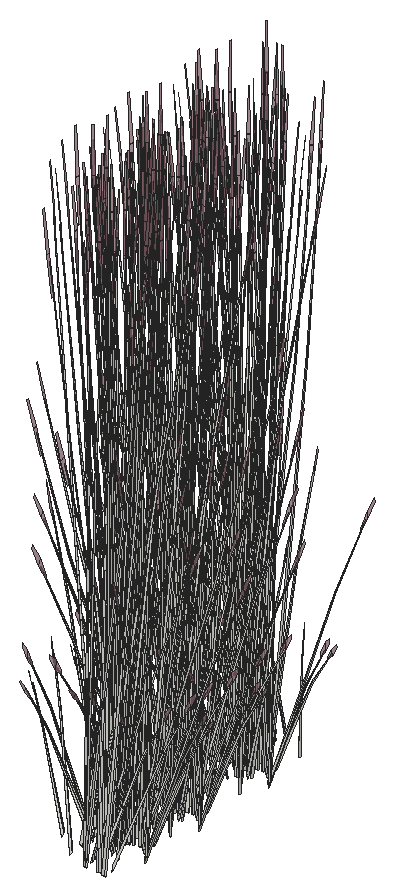
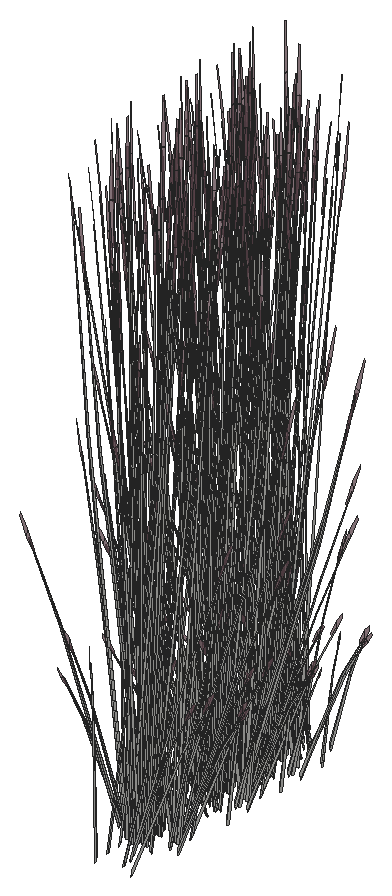
# SketchUp Ruby script. Lengths in inches.
U = 1.inch
M = Sketchup.active_model
def pt(a) = Geom::Point3d.new(a.map { |v| v * U })
def face(e, loops, mat)
  f = e.add_face(loops[0].map { |a| pt(a) })
  loops[1..].each { |l| e.add_face(l.map { |a| pt(a) }).erase! }
  f.material = f.back_material = mat if mat
  f
end
# faces: each face lists its corners as indices into pts; further lists are holes
def faces(e, pts, list, mat = nil) = list.each { |f| face(e, (f[0].is_a?(Array) ? f : [f]).map { |l| l.map { |i| pts[i] } }, mat) }
# xy, xz, yz: faces in a plane at the given z, y or x. An outline is a flat list of corners, or four numbers for a rectangle; further outlines are holes
def ring(l) = l.size == 4 ? [[l[0], l[1]], [l[2], l[1]], [l[2], l[3]], [l[0], l[3]]] : l.each_slice(2).to_a
def flat(e, list, mat, &to3) = list.each { |f| face(e, (f[0].is_a?(Array) ? f : [f]).map { |l| ring(l).map { |u, v| to3.(u, v) } }, mat) }
def xy(e, z, list, mat = nil) = flat(e, list, mat) { |x, y| [x, y, z] }
def xz(e, y, list, mat = nil) = flat(e, list, mat) { |x, z| [x, y, z] }
def yz(e, x, list, mat = nil) = flat(e, list, mat) { |y, z| [x, y, z] }
def lines(e, pts, list) = list.each { |a, b| e.add_line(pt(pts[a]), pt(pts[b])) }
# prism: a flat outline (further loops are holes) pulled along v
def prism(e, loops, v, mat = nil)
  f = face(e, loops, mat); d = Geom::Vector3d.new(v.map { |x| x * U })
  f.pushpull(f.normal.samedirection?(d) ? d.length : -d.length)
end
def box(e, o, s, mat = nil) = prism(e, [[o, [o[0] + s[0], o[1], o[2]], [o[0] + s[0], o[1] + s[1], o[2]], [o[0], o[1] + s[1], o[2]]]], [0, 0, s[2]], mat)
def at(x, y, z, deg = 0) = Geom::Transformation.translation(pt([x, y, z])) * Geom::Transformation.rotation(ORIGIN, Z_AXIS, deg.degrees)
def axes(o, x, y, z) = Geom::Transformation.new([*x, 0, *y, 0, *z, 0, *pt(o).to_a, 1])
def part(name) = M.definitions.add(name)
# library, detail: a bought-in or finely detailed component or shape, given as its bounding box
def library(name, o, s) = part(name).tap { |d| box(d.entities, o, s) }
def detail(e, o, s) = box(e.add_group.entities, o, s)
def put(e, d, t, mat = nil) = e.add_instance(d, t).tap { |i| i.material = mat if mat }
def group(e, t, mat = nil) = e.add_group.tap { |g| g.transformation = t; g.material = mat if mat }.entities
root = M.entities
M.materials.add("LightPink_Translucent").color = [144, 107, 117]
M.materials["LightPink_Translucent"].alpha = 0.75
c1 = part("blade")
p = [[2.15,0.21,22],[0,0.17,0],[0.09,0.45,0],[2.18,0.31,22],[2.29,0.31,22],[0.38,0.45,0],
  [2.48,0.24,33],[2.49,0.24,33],[2.48,0.22,33]]
faces(c1.entities,p,[[0,1,2,3],[4,5,2,3],[6,3,4,7],[8,0,3,6]])
c2 = part("seeds")
p = [[0.3,-0.1,1.38],[-0.01,-0.03,1.59],[-0.01,-0.03,0.03],[0.14,-0.07,-0.07],[0.29,-0.03,3],[0.15,0.01,3.11]]
faces(c2.entities,p,[[0,1,2,3],[1,0,4,5]],"LightPink_Translucent")
c3 = part("blade with seeds")
put(c3.entities,c1,at(0,0,0))
put(c3.entities,c2,axes([2.4,0.25,30.99],[1.5799,-0.05474,1.17369],[-0.12525,1.92788,0.29478],[-0.07173,-0.02425,1.56792]))
put(root,c3,axes([431.12,469.63,152.01],[0.51243,0,0],[0,0.52715,-0.43598],[0,0.12006,1.38303]))
put(root,c3,axes([430.91,469.9,151.86],[-0.51218,-0.00377,-0.04204],[0,-0.52715,0.42192],[-0.0161,0.12,1.33776]))
put(root,c3,axes([429.8,469.44,152.25],[0.46151,0.22505,-0.2458],[-0.22222,0.475,-0.42242],[0.0145,0.11662,1.34921]))
put(root,c3,axes([427.74,473.58,151.97],[-0.38118,0.39654,0.25983],[-0.38142,-0.39237,-0.30828],[-0.01331,-0.11261,1.39295]))
put(root,c3,axes([426.58,471.19,152.34],[0.17079,-0.21377,0.97034],[0.06739,0.33841,0.71294],[-0.12342,0.0606,0.21373]))
put(root,c3,axes([429.57,470.01,152.25],[0.04775,0.53819,-0.2458],[-0.49736,0.03254,-0.42242],[-0.08758,0.07169,1.34921]))
put(root,c3,axes([428.95,473.77,152.06],[0.46174,0.2286,0.2033],[-0.22222,0.475,0.42242],[0,-0.1095,1.35626]))
put(root,c3,axes([428.77,474.41,152.06],[0.10862,-0.55889,-0.19793],[0.515,0.09742,0.43313],[-0.08999,-0.07718,1.32161]))
put(root,c3,axes([426.95,473.17,152.34],[0.26163,-0.03375,0.97034],[-0.16596,0.29737,0.71294],[-0.12929,-0.04461,0.21373]))
put(root,c3,axes([428.8,473.45,152.3],[-0.44501,0.02912,0.37796],[-0.04024,-0.48332,-0.1819],[0.07967,-0.04899,1.2135]))
put(root,c3,axes([427.65,473.8,152.09],[0,0.47166,0.41945],[-0.45849,0,0],[0,-0.10742,1.33059]))
put(root,c3,axes([429.76,471.02,151.97],[0.51304,0.1533,0.25983],[-0.12835,0.54797,-0.30828],[-0.08491,0.06858,1.39295]))
put(root,c3,axes([430.27,472.16,152.01],[0.25622,-0.47263,0],[0.42866,0.26357,-0.43598],[0.09763,0.06003,1.38303]))
put(root,c3,axes([428.79,473.62,151.99],[0.17817,0.52741,0.38653],[-0.50909,0.1834,0.15168],[0.00622,-0.09691,1.34202]))
put(root,c3,axes([431.28,474.03,151.67],[-0.26394,0.0566,1.1961],[-0.04201,-0.45055,0.06846],[0.18486,-0.06819,0.68062]))
put(root,c3,axes([431.76,473.625,151.91],[-0.25407,-0.3016,-0.05481],[0.27826,-0.27635,-0.2485],[0.07884,-0.01946,0.81966]))
put(root,c3,axes([428.7,474.04,152.3],[-0.19883,0.425,0.37796],[-0.41314,-0.20454,-0.1819],[0,-0.09797,1.2135]))
put(root,c3,axes([430.42,470.97,152.34],[-0.23074,-0.13562,0.97034],[0.29794,-0.1378,0.71294],[0.08036,0.11673,0.21373]))
put(root,c3,axes([429.43,473.67,151.86],[0,-0.54574,0],[0.51243,0,0],[0,0,1.51605]))
put(root,c3,axes([430.05,472.4,152.09],[-0.38354,-0.23583,0.41945],[0.22925,-0.42288,0],[0.08735,0.05371,1.33059]))
put(root,c3,axes([430.8,474.0625,154.21],[0.3601,-0.20831,-0.60019],[0.20068,0.4288,0.07243],[0.17399,-0.04871,0.84903]))
put(root,c3,axes([429.18,473.32,151.99],[-0.33979,0.42804,0.38653],[-0.40368,-0.37784,0.15168],[0.08192,-0.04272,1.34202]))
put(root,c3,axes([430.08,471.3125,152],[0.25622,0.47263,0],[-0.42866,0.26357,-0.43598],[-0.09763,0.06003,1.38303]))
put(root,c3,axes([429.56,474.09,151.94],[-0.38118,-0.40596,-0.0518],[0.38142,-0.40621,0],[-0.01331,-0.01418,1.48322]))
put(root,c3,axes([430.48,471.47,151.26],[0.02986,-0.06809,1.48974],[0.37589,-0.20055,-0.22758],[0.11396,0.1038,0.25375]))
put(root,c3,axes([428.59,472.62,152.09],[-0.11838,0.46875,0.14904],[-0.43321,-0.13265,0.29641],[0.07483,-0.00228,1.35512]))
put(root,c3,axes([429.86,469.44,152.4],[-0.01119,-0.44408,1.19347],[0.50665,0.11511,0.50532],[-0.11983,0.243,1.12654]))
put(root,c3,axes([427.03,471.41,151.26],[0.05497,0.04712,1.48974],[0.09321,0.43661,-0.22758],[-0.12183,0.0931,0.25375]))
put(root,c3,axes([428.42,473,151.35],[-0.40337,0.18883,1.08919],[-0.12839,-0.54182,0.42321],[0.24769,0.00901,1.23883]))
put(root,c3,axes([429.5,473.14,152.21],[0.07906,-0.42093,0.12232],[0.38625,0.07307,-0.3493],[0.07029,0.04322,1.07074]))
put(root,c3,axes([428.83,474.14,151.99],[0.51796,0.09937,0.38653],[-0.10541,0.56124,0.15168],[-0.07569,-0.05419,1.34202]))
put(root,c3,axes([431.57,473.73,151.26],[-0.02142,-0.07161,1.48974],[0.14855,-0.41887,-0.22758],[0.14984,-0.00603,0.25375]))
put(root,c3,axes([427.14,473.66,151.26],[0.01039,0.07433,1.48974],[-0.20952,0.38819,-0.22758],[-0.14882,-0.01957,0.25375]))
put(root,c3,axes([429.33,473.25,152.3],[-0.24618,-0.39589,0.37796],[0.37289,-0.27878,-0.1819],[0.07967,0.04899,1.2135]))
put(root,c3,axes([430.46,471.59,152.25],[-0.26279,-0.01479,0.88755],[0.17355,-0.31417,0.49003],[0.10382,0.11162,0.6962]))
put(root,c3,axes([429.88,477.19,152.1875],[-0.11649,0.09547,1.20808],[-0.34886,-0.1671,-0.25981],[0.06467,-0.20781,0.51652]))
put(root,c3,axes([429.35,477.52,154.21],[-0.19559,-0.38351,-0.60019],[0.40262,-0.21373,0.07243],[-0.04574,-0.1853,0.84903]))
put(root,c3,axes([428.08,477.01,152.1875],[-0.02482,0.15429,1.20808],[-0.36278,0.12916,-0.25981],[-0.0848,-0.19943,0.51652]))
put(root,c3,axes([428.55,475.03,152.09],[0.44036,-0.12519,0.14904],[0.10874,0.46588,0.29641],[-0.03927,-0.06788,1.35512]))
put(root,c3,axes([429.46,473.27,152.25],[0.41376,-0.31314,-0.2458],[0.27514,0.44246,-0.42242],[0.10209,0.04493,1.34921]))
put(root,c3,axes([429.02,476.67,151.26],[-0.06874,0.01699,1.48974],[-0.38012,-0.19128,-0.22758],[0.00638,-0.15955,0.25375]))
put(root,c3,axes([429.78,473.79,151.86],[0.45849,0,0],[0,0.4883,0],[0,0,1.50718]))
put(root,c3,axes([430.17,477.9,154.21],[0.01066,-0.43628,-0.60019],[0.44902,0.0293,0.07243],[0.04739,-0.18483,0.84903]))
put(root,c3,axes([429,474.4,152.25],[-0.41376,0.31314,-0.2458],[-0.27514,-0.44246,-0.42242],[-0.10209,-0.04493,1.34921]))
put(root,c3,axes([429.6,470.82,152.1875],[0.00723,-0.15635,1.20808],[0.34559,-0.17464,-0.25981],[0.10668,0.18713,0.51652]))
put(root,c3,axes([429.91,472.64,152.09],[-0.44036,0.12519,0.14904],[-0.10874,-0.46588,0.29641],[0.03927,0.06788,1.35512]))
put(root,c3,axes([428.03,472.13,152.34],[-0.01061,-0.28045,0.97034],[0.26501,0.20003,0.71294],[-0.05212,0.13367,0.21373]))
put(root,c3,axes([429.46,476.43,152.34],[0.05257,0.27504,0.97034],[-0.29163,-0.15233,0.71294],[0.03138,-0.14083,0.21373]))
put(root,c3,axes([429.63,473.54,152.01],[-0.51796,-0.09937,0.41563],[0.10541,-0.56124,0.1631],[0.07569,0.05419,1.44303]))
put(root,c3,axes([429.21,474.92,151.86],[-0.13371,-0.40664,0],[0.38182,-0.1424,0],[0,0,1.30413]))
put(root,c3,axes([428.73,471.46,151.26],[0.06632,-0.02567,1.48974],[0.39894,0.14126,-0.22758],[0.01167,0.15921,0.25375]))
put(root,c3,axes([428.96,474.54,152.21],[-0.07906,0.42093,0.12232],[-0.38625,-0.07307,-0.3493],[-0.07029,-0.04322,1.07074]))
put(root,c3,axes([429.71,474.87,151.85],[0.43024,-0.16003,-0.16218],[0.15118,0.46099,0.00007],[0.04749,-0.01769,1.46908]))
put(root,c3,axes([429.86,475.06,152.09],[0.11838,-0.46875,0.14904],[0.43321,0.13265,0.29641],[-0.07483,0.00228,1.35512]))
put(root,c3,axes([429.77,474,151.87],[0.28606,0.30466,0],[-0.28606,0.30466,0],[0,0,1.42996]))
put(root,c3,axes([427.8125,471.52,152.38],[0.37228,-0.08352,0.05498],[0.08559,0.3365,-0.7291],[-0.0236,0.17034,0.65354]))
put(root,c3,axes([430.54,473.86,152.09],[-0.32198,-0.34356,0.14904],[0.32447,-0.33323,0.29641],[-0.03556,0.07016,1.35512]))
put(root,c3,axes([431.83,474.18,152.34],[-0.2532,0.07787,0.97034],[0.11918,-0.32181,0.71294],[0.13432,0.02202,0.21373]))
put(root,c3,axes([429.12,475.11,151.86],[-0.41314,-0.21175,0],[0.19883,-0.43999,0],[0,0,1.37455]))
put(root,c3,axes([429.46,474.55,152.08],[-0.40016,-0.37963,-0.21282],[0.33672,-0.42629,0.46574],[-0.10776,0.04441,1.42109]))
put(root,c3,axes([428.41,475.27,152.09],[0.38354,0.23583,0.41945],[-0.22925,0.42288,0],[-0.08735,-0.05371,1.33059]))
put(root,c3,axes([427.96,476.76,152.34],[0.21377,0.16416,0.97034],[-0.31132,0.09868,0.71294],[-0.06661,-0.12616,0.21373]))
put(root,c3,axes([428.47,477.63,154.21],[-0.34944,-0.22798,-0.60019],[0.24834,-0.39949,0.07243],[-0.1266,-0.13612,0.84903]))
put(root,c3,axes([429.76,473.64,152.3],[0.19883,-0.425,0.37796],[0.41314,0.20454,-0.1819],[0,0.09797,1.2135]))
put(root,c3,axes([429.68,473.88,151.9375],[0,0.54548,-0.04762],[-0.51243,0,0],[0,0.01714,1.5153]))
put(root,c3,axes([428.1875,475.52,152],[-0.25622,0.47263,0],[-0.42866,-0.26357,-0.43598],[-0.09763,-0.06003,1.38303]))
put(root,c3,axes([430.8,473.88,152.09],[0,-0.47166,0.41945],[0.45849,0,0],[0,0.10742,1.33059]))
put(root,c3,axes([427.79,477.26,151.26],[-0.0397,0.06213,1.48974],[-0.40116,0.13396,-0.22758],[-0.09691,-0.12186,0.25375]))
put(root,c3,axes([429.66,474.23,152.3],[0.44501,-0.02912,0.37796],[0.04024,0.48332,-0.1819],[-0.07967,0.04899,1.2135]))
put(root,c3,axes([429.93,473.74,152.21],[0.38182,-0.13755,0.12232],[0.13371,0.39278,-0.3493],[0,0.08644,1.07074]))
put(root,c3,axes([428.85,471.28,154.21],[0.19559,0.38351,-0.60019],[-0.40262,0.21373,0.07243],[0.04574,0.1853,0.84903]))
put(root,c3,axes([430.7,477.49,151.26],[-0.06134,-0.03716,1.48974],[-0.15755,-0.41512,-0.22758],[0.10629,-0.11265,0.25375]))
put(root,c3,axes([427.72,471.88,152.1875],[0.12932,-0.07441,1.20808],[0.31929,0.22435,-0.25981],[-0.09503,0.19413,0.51652]))
put(root,c3,axes([431.35,474.69,152.1875],[-0.0987,-0.116,1.20808],[0.12841,-0.38374,-0.25981],[0.19968,0.05198,0.51652]))
put(root,c3,axes([429.59,475.12,151.86],[0.41314,0.21175,0],[-0.19883,0.43999,0],[0,0,1.47801]))
put(root,c3,axes([429.75,475.59,151.85],[-0.25302,-0.47428,-0.04344],[0.42866,-0.26357,0.43598],[-0.10563,0.04516,1.38235]))
put(root,c3,axes([429.66,474.4375,152.21],[0.30276,0.28338,0.12232],[-0.25254,0.31972,-0.3493],[-0.07029,0.04322,1.07074]))
put(root,c3,axes([430.7,478.66,154.21],[0.21406,-0.37215,-0.60019],[0.37511,0.26448,0.07243],[0.12781,-0.13483,0.84903]))
put(root,c3,axes([428.38,477.57,152],[-0.25622,-0.47263,0],[0.42866,-0.26357,-0.43598],[0.09763,-0.06003,1.38303]))
put(root,c3,axes([428.95,477.01,151.8],[-0.28319,0.27058,-0.03288],[-0.25948,-0.29635,-0.1491],[-0.01827,-0.08397,0.4918]))
put(root,c3,axes([430.45,474.93,154.21],[0.40965,0.01136,-0.60019],[-0.02751,0.47821,0.07243],[0.17355,0.05047,0.84903]))
put(root,c3,axes([429.99,475.3125,152.09],[0.38354,-0.23583,0.41945],[0.22925,0.42288,0],[-0.08735,0.05371,1.33059]))
put(root,c3,axes([429.44,474.9375,151.9375],[0.17817,0.54185,-0.05079],[-0.50909,0.18987,0],[0.00622,0.01892,1.45452]))
put(root,c3,axes([426.88,474.69,152.1875],[0.14242,0.03872,1.20808],[0.09179,0.39548,-0.25981],[-0.19345,0.07403,0.51652]))
put(root,c3,axes([431.12,473.96,152.01],[0.51243,0,0],[0,0.52715,-0.43598],[0,0.12006,1.38303]))
put(root,c3,axes([430.91,474.23,151.86],[-0.51218,-0.00377,-0.04204],[0,-0.52715,0.42192],[-0.0161,0.12,1.33776]))
put(root,c3,axes([431.01,478.32,152.1875],[-0.1464,-0.01397,1.20808],[-0.14998,-0.37477,-0.25981],[0.17985,-0.10602,0.51652]))
put(root,c3,axes([429.8,473.77,152.25],[0.46151,0.22505,-0.2458],[-0.22222,0.475,-0.42242],[0.0145,0.11662,1.34921]))
put(root,c3,axes([426.58,475.52,152.34],[0.17079,-0.21377,0.97034],[0.06739,0.33841,0.71294],[-0.12342,0.0606,0.21373]))
put(root,c3,axes([429.57,474.33,152.25],[0.04775,0.53819,-0.2458],[-0.49736,0.03254,-0.42242],[-0.08758,0.07169,1.34921]))
put(root,c3,axes([431.18,477.63,152.34],[-0.1365,0.2401,0.97034],[-0.11733,-0.32258,0.71294],[0.11274,-0.08083,0.21373]))
put(root,c3,axes([428.89,478.88,152.25],[-0.04775,-0.53819,-0.2458],[0.49736,-0.03254,-0.42242],[0.08758,-0.07169,1.34921]))
put(root,c3,axes([427.54,477.5,151.8],[-0.11822,0.38513,-0.03288],[-0.36385,-0.11847,-0.1491],[-0.05524,-0.06299,0.4918]))
put(root,c3,axes([428.66,479.44,152.25],[-0.46151,-0.22505,-0.2458],[0.22222,-0.475,-0.42242],[-0.0145,-0.11662,1.34921]))
put(root,c3,axes([429.76,475.34,151.97],[0.51304,0.1533,0.25983],[-0.12835,0.54797,-0.30828],[-0.08491,0.06858,1.39295]))
put(root,c3,axes([427.34,479.26,152],[-0.51243,0,0],[0,-0.52715,-0.43598],[0,-0.12006,1.38303]))
put(root,c3,axes([427.43,478.3125,152.1875],[0.08001,0.13132,1.20808],[-0.18437,0.35694,-0.25981],[-0.18931,-0.08532,0.51652]))
put(root,c3,axes([427.76,478.2,154.21],[-0.40965,-0.01136,-0.60019],[0.02751,-0.47821,0.07243],[-0.17355,-0.05047,0.84903]))
put(root,c3,axes([430.42,475.29,152.34],[-0.23074,-0.13562,0.97034],[0.29794,-0.1378,0.71294],[0.08036,0.11673,0.21373]))
put(root,c3,axes([430.08,475.64,152],[0.25622,0.47263,0],[-0.42866,0.26357,-0.43598],[-0.09763,0.06003,1.38303]))
put(root,c3,axes([430.48,475.8,151.26],[0.02986,-0.06809,1.48974],[0.37589,-0.20055,-0.22758],[0.11396,0.1038,0.25375]))
put(root,c3,axes([429.86,473.77,152.4],[-0.01119,-0.44408,1.19347],[0.50665,0.11511,0.50532],[-0.11983,0.243,1.12654]))
put(root,c3,axes([427.74,479.12,151.97],[-0.38118,0.39654,0.25983],[-0.38142,-0.39237,-0.30828],[-0.01331,-0.11261,1.39295]))
put(root,c3,axes([427.03,475.74,151.26],[0.05497,0.04712,1.48974],[0.09321,0.43661,-0.22758],[-0.12183,0.0931,0.25375]))
put(root,c3,axes([428.95,479.3,152.06],[0.46174,0.2286,0.2033],[-0.22222,0.475,0.42242],[0,-0.1095,1.35626]))
put(root,c3,axes([428.77,479.94,152.06],[0.10862,-0.55889,-0.19793],[0.515,0.09742,0.43313],[-0.08999,-0.07718,1.32161]))
put(root,c3,axes([430.46,475.91,152.25],[-0.26279,-0.01479,0.88755],[0.17355,-0.31417,0.49003],[0.10382,0.11162,0.6962]))
put(root,c3,axes([426.95,478.71,152.34],[0.26163,-0.03375,0.97034],[-0.16596,0.29737,0.71294],[-0.12929,-0.04461,0.21373]))
put(root,c3,axes([428.8,478.98,152.3],[-0.44501,0.02912,0.37796],[-0.04024,-0.48332,-0.1819],[0.07967,-0.04899,1.2135]))
put(root,c3,axes([427.65,479.34,152.09],[0,0.47166,0.41945],[-0.45849,0,0],[0,-0.10742,1.33059]))
put(root,c3,axes([430.27,477.69,152.01],[0.25622,-0.47263,0],[0.42866,0.26357,-0.43598],[0.09763,0.06003,1.38303]))
put(root,c3,axes([428.79,479.16,151.99],[0.17817,0.52741,0.38653],[-0.50909,0.1834,0.15168],[0.00622,-0.09691,1.34202]))
put(root,c3,axes([429.6,475.15,152.1875],[0.00723,-0.15635,1.20808],[0.34559,-0.17464,-0.25981],[0.10668,0.18713,0.51652]))
put(root,c3,axes([431.28,479.5625,151.67],[-0.26394,0.0566,1.1961],[-0.04201,-0.45055,0.06846],[0.18486,-0.06819,0.68062]))
put(root,c3,axes([431.76,479.16,151.91],[-0.25407,-0.3016,-0.05481],[0.27826,-0.27635,-0.2485],[0.07884,-0.01946,0.81966]))
put(root,c3,axes([428.7,479.57,152.3],[-0.19883,0.425,0.37796],[-0.41314,-0.20454,-0.1819],[0,-0.09797,1.2135]))
put(root,c3,axes([429.43,479.2,151.86],[0,-0.54574,0],[0.51243,0,0],[0,0,1.51605]))
put(root,c3,axes([430.05,477.94,152.09],[-0.38354,-0.23583,0.41945],[0.22925,-0.42288,0],[0.08735,0.05371,1.33059]))
put(root,c3,axes([430.8,479.6,154.21],[0.3601,-0.20831,-0.60019],[0.20068,0.4288,0.07243],[0.17399,-0.04871,0.84903]))
put(root,c3,axes([428.03,476.45,152.34],[-0.01061,-0.28045,0.97034],[0.26501,0.20003,0.71294],[-0.05212,0.13367,0.21373]))
put(root,c3,axes([429.18,478.86,151.99],[-0.33979,0.42804,0.38653],[-0.40368,-0.37784,0.15168],[0.08192,-0.04272,1.34202]))
put(root,c3,axes([428.73,475.78,151.26],[0.06632,-0.02567,1.48974],[0.39894,0.14126,-0.22758],[0.01167,0.15921,0.25375]))
put(root,c3,axes([429.56,479.625,151.94],[-0.38118,-0.40596,-0.0518],[0.38142,-0.40621,0],[-0.01331,-0.01418,1.48322]))
put(root,c3,axes([428.59,478.15,152.09],[-0.11838,0.46875,0.14904],[-0.43321,-0.13265,0.29641],[0.07483,-0.00228,1.35512]))
put(root,c3,axes([428.42,478.53,151.35],[-0.40337,0.18883,1.08919],[-0.12839,-0.54182,0.42321],[0.24769,0.00901,1.23883]))
put(root,c3,axes([429.5,478.67,152.21],[0.07906,-0.42093,0.12232],[0.38625,0.07307,-0.3493],[0.07029,0.04322,1.07074]))
put(root,c3,axes([427.8125,475.85,152.38],[0.37228,-0.08352,0.05498],[0.08559,0.3365,-0.7291],[-0.0236,0.17034,0.65354]))
put(root,c3,axes([428.83,479.67,151.99],[0.51796,0.09937,0.38653],[-0.10541,0.56124,0.15168],[-0.07569,-0.05419,1.34202]))
put(root,c3,axes([431.57,479.27,151.26],[-0.02142,-0.07161,1.48974],[0.14855,-0.41887,-0.22758],[0.14984,-0.00603,0.25375]))
put(root,c3,axes([427.14,479.19,151.26],[0.01039,0.07433,1.48974],[-0.20952,0.38819,-0.22758],[-0.14882,-0.01957,0.25375]))
put(root,c3,axes([429.33,478.78,152.3],[-0.24618,-0.39589,0.37796],[0.37289,-0.27878,-0.1819],[0.07967,0.04899,1.2135]))
put(root,c3,axes([428.55,480.57,152.09],[0.44036,-0.12519,0.14904],[0.10874,0.46588,0.29641],[-0.03927,-0.06788,1.35512]))
put(root,c3,axes([429.46,478.8125,152.25],[0.41376,-0.31314,-0.2458],[0.27514,0.44246,-0.42242],[0.10209,0.04493,1.34921]))
put(root,c3,axes([429.78,479.32,151.86],[0.45849,0,0],[0,0.4883,0],[0,0,1.50718]))
put(root,c3,axes([429,479.9375,152.25],[-0.41376,0.31314,-0.2458],[-0.27514,-0.44246,-0.42242],[-0.10209,-0.04493,1.34921]))
put(root,c3,axes([429.91,478.18,152.09],[-0.44036,0.12519,0.14904],[-0.10874,-0.46588,0.29641],[0.03927,0.06788,1.35512]))
put(root,c3,axes([428.85,475.6,154.21],[0.19559,0.38351,-0.60019],[-0.40262,0.21373,0.07243],[0.04574,0.1853,0.84903]))
put(root,c3,axes([427.72,476.2,152.1875],[0.12932,-0.07441,1.20808],[0.31929,0.22435,-0.25981],[-0.09503,0.19413,0.51652]))
put(root,c3,axes([429.63,479.07,152.01],[-0.51796,-0.09937,0.41563],[0.10541,-0.56124,0.1631],[0.07569,0.05419,1.44303]))
put(root,c3,axes([429.21,480.46,151.86],[-0.13371,-0.40664,0],[0.38182,-0.1424,0],[0,0,1.30413]))
put(root,c3,axes([428.96,480.07,152.21],[-0.07906,0.42093,0.12232],[-0.38625,-0.07307,-0.3493],[-0.07029,-0.04322,1.07074]))
put(root,c3,axes([429.71,480.4,151.85],[0.43024,-0.16003,-0.16218],[0.15118,0.46099,0.00007],[0.04749,-0.01769,1.46908]))
put(root,c3,axes([429.86,480.6,152.09],[0.11838,-0.46875,0.14904],[0.43321,0.13265,0.29641],[-0.07483,0.00228,1.35512]))
put(root,c3,axes([429.77,479.53,151.87],[0.28606,0.30466,0],[-0.28606,0.30466,0],[0,0,1.42996]))
put(root,c3,axes([430.54,479.4,152.09],[-0.32198,-0.34356,0.14904],[0.32447,-0.33323,0.29641],[-0.03556,0.07016,1.35512]))
put(root,c3,axes([431.83,479.71,152.34],[-0.2532,0.07787,0.97034],[0.11918,-0.32181,0.71294],[0.13432,0.02202,0.21373]))
put(root,c3,axes([429.12,480.64,151.86],[-0.41314,-0.21175,0],[0.19883,-0.43999,0],[0,0,1.37455]))
put(root,c3,axes([429.46,480.08,152.08],[-0.40016,-0.37963,-0.21282],[0.33672,-0.42629,0.46574],[-0.10776,0.04441,1.42109]))
put(root,c3,axes([428.41,480.81,152.09],[0.38354,0.23583,0.41945],[-0.22925,0.42288,0],[-0.08735,-0.05371,1.33059]))
put(root,c3,axes([429.76,479.18,152.3],[0.19883,-0.425,0.37796],[0.41314,0.20454,-0.1819],[0,0.09797,1.2135]))
put(root,c3,axes([429.68,479.42,151.9375],[0,0.54548,-0.04762],[-0.51243,0,0],[0,0.01714,1.5153]))
put(root,c3,axes([428.1875,481.06,152],[-0.25622,0.47263,0],[-0.42866,-0.26357,-0.43598],[-0.09763,-0.06003,1.38303]))
put(root,c3,axes([430.8,479.41,152.09],[0,-0.47166,0.41945],[0.45849,0,0],[0,0.10742,1.33059]))
put(root,c3,axes([429.66,479.77,152.3],[0.44501,-0.02912,0.37796],[0.04024,0.48332,-0.1819],[-0.07967,0.04899,1.2135]))
put(root,c3,axes([429.93,479.27,152.21],[0.38182,-0.13755,0.12232],[0.13371,0.39278,-0.3493],[0,0.08644,1.07074]))
put(root,c3,axes([429.88,484.41,152.1875],[-0.11649,0.09547,1.20808],[-0.34886,-0.1671,-0.25981],[0.06467,-0.20781,0.51652]))
put(root,c3,axes([428.08,484.23,152.1875],[-0.02482,0.15429,1.20808],[-0.36278,0.12916,-0.25981],[-0.0848,-0.19943,0.51652]))
put(root,c3,axes([431.35,480.23,152.1875],[-0.0987,-0.116,1.20808],[0.12841,-0.38374,-0.25981],[0.19968,0.05198,0.51652]))
put(root,c3,axes([429.02,483.89,151.26],[-0.06874,0.01699,1.48974],[-0.38012,-0.19128,-0.22758],[0.00638,-0.15955,0.25375]))
put(root,c3,axes([429.59,480.65,151.86],[0.41314,0.21175,0],[-0.19883,0.43999,0],[0,0,1.47801]))
put(root,c3,axes([429.75,481.12,151.85],[-0.25302,-0.47428,-0.04344],[0.42866,-0.26357,0.43598],[-0.10563,0.04516,1.38235]))
put(root,c3,axes([429.66,479.97,152.21],[0.30276,0.28338,0.12232],[-0.25254,0.31972,-0.3493],[-0.07029,0.04322,1.07074]))
put(root,c3,axes([429.46,483.65,152.34],[0.05257,0.27504,0.97034],[-0.29163,-0.15233,0.71294],[0.03138,-0.14083,0.21373]))
put(root,c3,axes([430.45,480.46,154.21],[0.40965,0.01136,-0.60019],[-0.02751,0.47821,0.07243],[0.17355,0.05047,0.84903]))
put(root,c3,axes([429.99,480.85,152.09],[0.38354,-0.23583,0.41945],[0.22925,0.42288,0],[-0.08735,0.05371,1.33059]))
put(root,c3,axes([429.44,480.47,151.9375],[0.17817,0.54185,-0.05079],[-0.50909,0.18987,0],[0.00622,0.01892,1.45452]))
put(root,c3,axes([426.88,480.23,152.1875],[0.14242,0.03872,1.20808],[0.09179,0.39548,-0.25981],[-0.19345,0.07403,0.51652]))
put(root,c3,axes([431.12,479.49,152.01],[0.51243,0,0],[0,0.52715,-0.43598],[0,0.12006,1.38303]))
put(root,c3,axes([430.91,479.76,151.86],[-0.51218,-0.00377,-0.04204],[0,-0.52715,0.42192],[-0.0161,0.12,1.33776]))
put(root,c3,axes([429.8,479.31,152.25],[0.46151,0.22505,-0.2458],[-0.22222,0.475,-0.42242],[0.0145,0.11662,1.34921]))
put(root,c3,axes([426.58,481.06,152.34],[0.17079,-0.21377,0.97034],[0.06739,0.33841,0.71294],[-0.12342,0.0606,0.21373]))
put(root,c3,axes([427.96,483.98,152.34],[0.21377,0.16416,0.97034],[-0.31132,0.09868,0.71294],[-0.06661,-0.12616,0.21373]))
put(root,c3,axes([429.57,479.87,152.25],[0.04775,0.53819,-0.2458],[-0.49736,0.03254,-0.42242],[-0.08758,0.07169,1.34921]))
put(root,c3,axes([428.47,484.85,154.21],[-0.34944,-0.22798,-0.60019],[0.24834,-0.39949,0.07243],[-0.1266,-0.13612,0.84903]))
put(root,c3,axes([427.79,484.47,151.26],[-0.0397,0.06213,1.48974],[-0.40116,0.13396,-0.22758],[-0.09691,-0.12186,0.25375]))
put(root,c3,axes([429.76,480.88,151.97],[0.51304,0.1533,0.25983],[-0.12835,0.54797,-0.30828],[-0.08491,0.06858,1.39295]))
put(root,c3,axes([430.7,484.7,151.26],[-0.06134,-0.03716,1.48974],[-0.15755,-0.41512,-0.22758],[0.10629,-0.11265,0.25375]))
put(root,c3,axes([430.42,480.83,152.34],[-0.23074,-0.13562,0.97034],[0.29794,-0.1378,0.71294],[0.08036,0.11673,0.21373]))
put(root,c3,axes([428.38,484.79,152],[-0.25622,-0.47263,0],[0.42866,-0.26357,-0.43598],[0.09763,-0.06003,1.38303]))
put(root,c3,axes([430.08,481.17,152],[0.25622,0.47263,0],[-0.42866,0.26357,-0.43598],[-0.09763,0.06003,1.38303]))
put(root,c3,axes([428.95,484.22,151.8],[-0.28319,0.27058,-0.03288],[-0.25948,-0.29635,-0.1491],[-0.01827,-0.08397,0.4918]))
put(root,c3,axes([430.48,481.33,151.26],[0.02986,-0.06809,1.48974],[0.37589,-0.20055,-0.22758],[0.11396,0.1038,0.25375]))
put(root,c3,axes([429.86,479.3,152.4],[-0.01119,-0.44408,1.19347],[0.50665,0.11511,0.50532],[-0.11983,0.243,1.12654]))
put(root,c3,axes([427.03,481.28,151.26],[0.05497,0.04712,1.48974],[0.09321,0.43661,-0.22758],[-0.12183,0.0931,0.25375]))
put(root,c3,axes([430.46,481.45,152.25],[-0.26279,-0.01479,0.88755],[0.17355,-0.31417,0.49003],[0.10382,0.11162,0.6962]))
put(root,c3,axes([431.01,485.53,152.1875],[-0.1464,-0.01397,1.20808],[-0.14998,-0.37477,-0.25981],[0.17985,-0.10602,0.51652]))
put(root,c3,axes([431.18,484.84,152.34],[-0.1365,0.2401,0.97034],[-0.11733,-0.32258,0.71294],[0.11274,-0.08083,0.21373]))
put(root,c3,axes([429.6,480.69,152.1875],[0.00723,-0.15635,1.20808],[0.34559,-0.17464,-0.25981],[0.10668,0.18713,0.51652]))
put(root,c3,axes([428.89,486.09,152.25],[-0.04775,-0.53819,-0.2458],[0.49736,-0.03254,-0.42242],[0.08758,-0.07169,1.34921]))
put(root,c3,axes([428.03,481.99,152.34],[-0.01061,-0.28045,0.97034],[0.26501,0.20003,0.71294],[-0.05212,0.13367,0.21373]))
put(root,c3,axes([427.54,484.71,151.8],[-0.11822,0.38513,-0.03288],[-0.36385,-0.11847,-0.1491],[-0.05524,-0.06299,0.4918]))
put(root,c3,axes([428.66,486.66,152.25],[-0.46151,-0.22505,-0.2458],[0.22222,-0.475,-0.42242],[-0.0145,-0.11662,1.34921]))
put(root,c3,axes([427.34,486.47,152],[-0.51243,0,0],[0,-0.52715,-0.43598],[0,-0.12006,1.38303]))
put(root,c3,axes([428.73,481.32,151.26],[0.06632,-0.02567,1.48974],[0.39894,0.14126,-0.22758],[0.01167,0.15921,0.25375]))
put(root,c3,axes([427.43,485.53,152.1875],[0.08001,0.13132,1.20808],[-0.18437,0.35694,-0.25981],[-0.18931,-0.08532,0.51652]))
put(root,c3,axes([427.8125,481.38,152.38],[0.37228,-0.08352,0.05498],[0.08559,0.3365,-0.7291],[-0.0236,0.17034,0.65354]))
put(root,c3,axes([427.74,486.33,151.97],[-0.38118,0.39654,0.25983],[-0.38142,-0.39237,-0.30828],[-0.01331,-0.11261,1.39295]))
put(root,c3,axes([428.95,486.51,152.06],[0.46174,0.2286,0.2033],[-0.22222,0.475,0.42242],[0,-0.1095,1.35626]))
put(root,c3,axes([428.77,487.16,152.06],[0.10862,-0.55889,-0.19793],[0.515,0.09742,0.43313],[-0.08999,-0.07718,1.32161]))
put(root,c3,axes([428.85,481.14,154.21],[0.19559,0.38351,-0.60019],[-0.40262,0.21373,0.07243],[0.04574,0.1853,0.84903]))
put(root,c3,axes([426.95,485.92,152.34],[0.26163,-0.03375,0.97034],[-0.16596,0.29737,0.71294],[-0.12929,-0.04461,0.21373]))
put(root,c3,axes([427.72,481.74,152.1875],[0.12932,-0.07441,1.20808],[0.31929,0.22435,-0.25981],[-0.09503,0.19413,0.51652]))
put(root,c3,axes([428.8,486.2,152.3],[-0.44501,0.02912,0.37796],[-0.04024,-0.48332,-0.1819],[0.07967,-0.04899,1.2135]))
put(root,c3,axes([427.65,486.55,152.09],[0,0.47166,0.41945],[-0.45849,0,0],[0,-0.10742,1.33059]))
put(root,c3,axes([430.27,484.91,152.01],[0.25622,-0.47263,0],[0.42866,0.26357,-0.43598],[0.09763,0.06003,1.38303]))
put(root,c3,axes([428.79,486.37,151.99],[0.17817,0.52741,0.38653],[-0.50909,0.1834,0.15168],[0.00622,-0.09691,1.34202]))
put(root,c3,axes([431.28,486.78,151.67],[-0.26394,0.0566,1.1961],[-0.04201,-0.45055,0.06846],[0.18486,-0.06819,0.68062]))
put(root,c3,axes([431.76,486.375,151.91],[-0.25407,-0.3016,-0.05481],[0.27826,-0.27635,-0.2485],[0.07884,-0.01946,0.81966]))
put(root,c3,axes([428.7,486.79,152.3],[-0.19883,0.425,0.37796],[-0.41314,-0.20454,-0.1819],[0,-0.09797,1.2135]))
put(root,c3,axes([429.43,486.42,151.86],[0,-0.54574,0],[0.51243,0,0],[0,0,1.51605]))
put(root,c3,axes([430.05,485.15,152.09],[-0.38354,-0.23583,0.41945],[0.22925,-0.42288,0],[0.08735,0.05371,1.33059]))
put(root,c3,axes([429.18,486.07,151.99],[-0.33979,0.42804,0.38653],[-0.40368,-0.37784,0.15168],[0.08192,-0.04272,1.34202]))
put(root,c3,axes([429.56,486.84,151.94],[-0.38118,-0.40596,-0.0518],[0.38142,-0.40621,0],[-0.01331,-0.01418,1.48322]))
put(root,c3,axes([428.59,485.37,152.09],[-0.11838,0.46875,0.14904],[-0.43321,-0.13265,0.29641],[0.07483,-0.00228,1.35512]))
put(root,c3,axes([428.42,485.74,151.35],[-0.40337,0.18883,1.08919],[-0.12839,-0.54182,0.42321],[0.24769,0.00901,1.23883]))
put(root,c3,axes([429.5,485.89,152.21],[0.07906,-0.42093,0.12232],[0.38625,0.07307,-0.3493],[0.07029,0.04322,1.07074]))
put(root,c3,axes([428.83,486.89,151.99],[0.51796,0.09937,0.38653],[-0.10541,0.56124,0.15168],[-0.07569,-0.05419,1.34202]))
put(root,c3,axes([431.57,486.48,151.26],[-0.02142,-0.07161,1.48974],[0.14855,-0.41887,-0.22758],[0.14984,-0.00603,0.25375]))
put(root,c3,axes([427.14,486.41,151.26],[0.01039,0.07433,1.48974],[-0.20952,0.38819,-0.22758],[-0.14882,-0.01957,0.25375]))
put(root,c3,axes([429.33,486,152.3],[-0.24618,-0.39589,0.37796],[0.37289,-0.27878,-0.1819],[0.07967,0.04899,1.2135]))
put(root,c3,axes([428.55,487.78,152.09],[0.44036,-0.12519,0.14904],[0.10874,0.46588,0.29641],[-0.03927,-0.06788,1.35512]))
put(root,c3,axes([429.46,486.02,152.25],[0.41376,-0.31314,-0.2458],[0.27514,0.44246,-0.42242],[0.10209,0.04493,1.34921]))
put(root,c3,axes([429.78,486.54,151.86],[0.45849,0,0],[0,0.4883,0],[0,0,1.50718]))
put(root,c3,axes([429,487.15,152.25],[-0.41376,0.31314,-0.2458],[-0.27514,-0.44246,-0.42242],[-0.10209,-0.04493,1.34921]))
put(root,c3,axes([429.91,485.39,152.09],[-0.44036,0.12519,0.14904],[-0.10874,-0.46588,0.29641],[0.03927,0.06788,1.35512]))
put(root,c3,axes([429.88,490.57,152.1875],[-0.11649,0.09547,1.20808],[-0.34886,-0.1671,-0.25981],[0.06467,-0.20781,0.51652]))
put(root,c3,axes([429.63,486.29,152.01],[-0.51796,-0.09937,0.41563],[0.10541,-0.56124,0.1631],[0.07569,0.05419,1.44303]))
put(root,c3,axes([428.08,490.39,152.1875],[-0.02482,0.15429,1.20808],[-0.36278,0.12916,-0.25981],[-0.0848,-0.19943,0.51652]))
put(root,c3,axes([429.21,487.67,151.86],[-0.13371,-0.40664,0],[0.38182,-0.1424,0],[0,0,1.30413]))
put(root,c3,axes([428.96,487.29,152.21],[-0.07906,0.42093,0.12232],[-0.38625,-0.07307,-0.3493],[-0.07029,-0.04322,1.07074]))
put(root,c3,axes([429.02,490.05,151.26],[-0.06874,0.01699,1.48974],[-0.38012,-0.19128,-0.22758],[0.00638,-0.15955,0.25375]))
put(root,c3,axes([429.71,487.62,151.85],[0.43024,-0.16003,-0.16218],[0.15118,0.46099,0.00007],[0.04749,-0.01769,1.46908]))
put(root,c3,axes([429.86,487.81,152.09],[0.11838,-0.46875,0.14904],[0.43321,0.13265,0.29641],[-0.07483,0.00228,1.35512]))
put(root,c3,axes([429.77,486.75,151.87],[0.28606,0.30466,0],[-0.28606,0.30466,0],[0,0,1.42996]))
put(root,c3,axes([430.54,486.61,152.09],[-0.32198,-0.34356,0.14904],[0.32447,-0.33323,0.29641],[-0.03556,0.07016,1.35512]))
put(root,c3,axes([431.83,486.93,152.34],[-0.2532,0.07787,0.97034],[0.11918,-0.32181,0.71294],[0.13432,0.02202,0.21373]))
put(root,c3,axes([429.12,487.86,151.86],[-0.41314,-0.21175,0],[0.19883,-0.43999,0],[0,0,1.37455]))
put(root,c3,axes([429.46,487.29,152.08],[-0.40016,-0.37963,-0.21282],[0.33672,-0.42629,0.46574],[-0.10776,0.04441,1.42109]))
put(root,c3,axes([428.41,488.02,152.09],[0.38354,0.23583,0.41945],[-0.22925,0.42288,0],[-0.08735,-0.05371,1.33059]))
put(root,c3,axes([429.76,486.39,152.3],[0.19883,-0.425,0.37796],[0.41314,0.20454,-0.1819],[0,0.09797,1.2135]))
put(root,c3,axes([429.46,489.8125,152.34],[0.05257,0.27504,0.97034],[-0.29163,-0.15233,0.71294],[0.03138,-0.14083,0.21373]))
put(root,c3,axes([429.68,486.63,151.9375],[0,0.54548,-0.04762],[-0.51243,0,0],[0,0.01714,1.5153]))
put(root,c3,axes([428.1875,488.27,152],[-0.25622,0.47263,0],[-0.42866,-0.26357,-0.43598],[-0.09763,-0.06003,1.38303]))
put(root,c3,axes([430.8,486.625,152.09],[0,-0.47166,0.41945],[0.45849,0,0],[0,0.10742,1.33059]))
put(root,c3,axes([429.66,486.98,152.3],[0.44501,-0.02912,0.37796],[0.04024,0.48332,-0.1819],[-0.07967,0.04899,1.2135]))
put(root,c3,axes([429.93,486.49,152.21],[0.38182,-0.13755,0.12232],[0.13371,0.39278,-0.3493],[0,0.08644,1.07074]))
put(root,c3,axes([427.96,490.14,152.34],[0.21377,0.16416,0.97034],[-0.31132,0.09868,0.71294],[-0.06661,-0.12616,0.21373]))
put(root,c3,axes([431.35,487.44,152.1875],[-0.0987,-0.116,1.20808],[0.12841,-0.38374,-0.25981],[0.19968,0.05198,0.51652]))
put(root,c3,axes([429.59,487.87,151.86],[0.41314,0.21175,0],[-0.19883,0.43999,0],[0,0,1.47801]))
put(root,c3,axes([429.75,488.33,151.85],[-0.25302,-0.47428,-0.04344],[0.42866,-0.26357,0.43598],[-0.10563,0.04516,1.38235]))
put(root,c3,axes([429.66,487.1875,152.21],[0.30276,0.28338,0.12232],[-0.25254,0.31972,-0.3493],[-0.07029,0.04322,1.07074]))
put(root,c3,axes([427.79,490.64,151.26],[-0.0397,0.06213,1.48974],[-0.40116,0.13396,-0.22758],[-0.09691,-0.12186,0.25375]))
put(root,c3,axes([430.7,490.87,151.26],[-0.06134,-0.03716,1.48974],[-0.15755,-0.41512,-0.22758],[0.10629,-0.11265,0.25375]))
put(root,c3,axes([429.99,488.0625,152.09],[0.38354,-0.23583,0.41945],[0.22925,0.42288,0],[-0.08735,0.05371,1.33059]))
put(root,c3,axes([429.44,487.6875,151.9375],[0.17817,0.54185,-0.05079],[-0.50909,0.18987,0],[0.00622,0.01892,1.45452]))
put(root,c3,axes([426.88,487.44,152.1875],[0.14242,0.03872,1.20808],[0.09179,0.39548,-0.25981],[-0.19345,0.07403,0.51652]))
put(root,c3,axes([431.12,486.71,152.01],[0.51243,0,0],[0,0.52715,-0.43598],[0,0.12006,1.38303]))
put(root,c3,axes([430.91,486.98,151.86],[-0.51218,-0.00377,-0.04204],[0,-0.52715,0.42192],[-0.0161,0.12,1.33776]))
put(root,c3,axes([429.8,486.52,152.25],[0.46151,0.22505,-0.2458],[-0.22222,0.475,-0.42242],[0.0145,0.11662,1.34921]))
